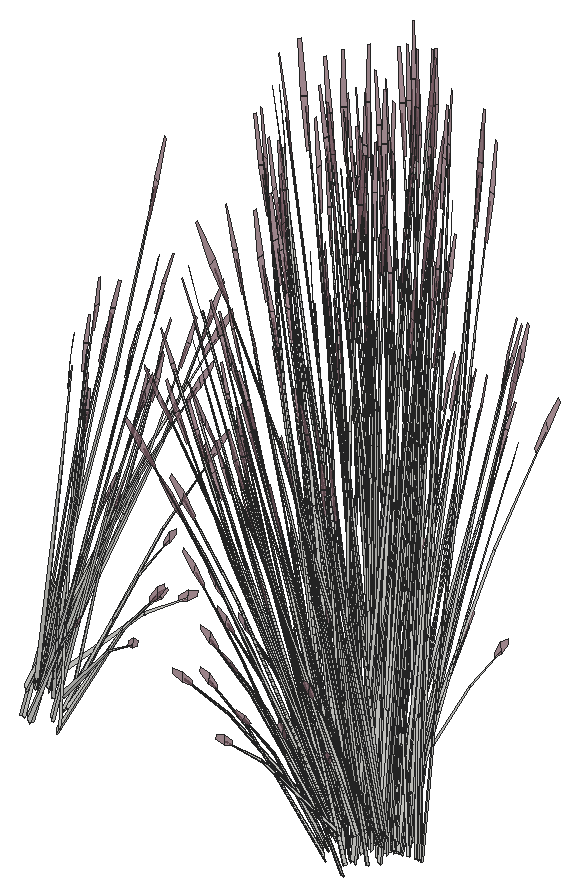
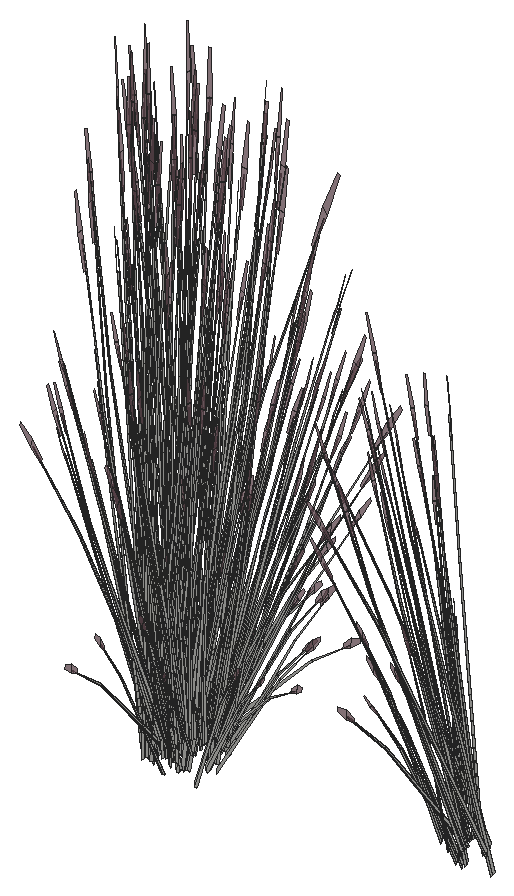
# SketchUp Ruby script. Lengths in inches.
U = 1.inch
M = Sketchup.active_model
def pt(a) = Geom::Point3d.new(a.map { |v| v * U })
def face(e, loops, mat)
  f = e.add_face(loops[0].map { |a| pt(a) })
  loops[1..].each { |l| e.add_face(l.map { |a| pt(a) }).erase! }
  f.material = f.back_material = mat if mat
  f
end
# faces: each face lists its corners as indices into pts; further lists are holes
def faces(e, pts, list, mat = nil) = list.each { |f| face(e, (f[0].is_a?(Array) ? f : [f]).map { |l| l.map { |i| pts[i] } }, mat) }
# xy, xz, yz: faces in a plane at the given z, y or x. An outline is a flat list of corners, or four numbers for a rectangle; further outlines are holes
def ring(l) = l.size == 4 ? [[l[0], l[1]], [l[2], l[1]], [l[2], l[3]], [l[0], l[3]]] : l.each_slice(2).to_a
def flat(e, list, mat, &to3) = list.each { |f| face(e, (f[0].is_a?(Array) ? f : [f]).map { |l| ring(l).map { |u, v| to3.(u, v) } }, mat) }
def xy(e, z, list, mat = nil) = flat(e, list, mat) { |x, y| [x, y, z] }
def xz(e, y, list, mat = nil) = flat(e, list, mat) { |x, z| [x, y, z] }
def yz(e, x, list, mat = nil) = flat(e, list, mat) { |y, z| [x, y, z] }
def lines(e, pts, list) = list.each { |a, b| e.add_line(pt(pts[a]), pt(pts[b])) }
# prism: a flat outline (further loops are holes) pulled along v
def prism(e, loops, v, mat = nil)
  f = face(e, loops, mat); d = Geom::Vector3d.new(v.map { |x| x * U })
  f.pushpull(f.normal.samedirection?(d) ? d.length : -d.length)
end
def box(e, o, s, mat = nil) = prism(e, [[o, [o[0] + s[0], o[1], o[2]], [o[0] + s[0], o[1] + s[1], o[2]], [o[0], o[1] + s[1], o[2]]]], [0, 0, s[2]], mat)
def at(x, y, z, deg = 0) = Geom::Transformation.translation(pt([x, y, z])) * Geom::Transformation.rotation(ORIGIN, Z_AXIS, deg.degrees)
def axes(o, x, y, z) = Geom::Transformation.new([*x, 0, *y, 0, *z, 0, *pt(o).to_a, 1])
def part(name) = M.definitions.add(name)
# library, detail: a bought-in or finely detailed component or shape, given as its bounding box
def library(name, o, s) = part(name).tap { |d| box(d.entities, o, s) }
def detail(e, o, s) = box(e.add_group.entities, o, s)
def put(e, d, t, mat = nil) = e.add_instance(d, t).tap { |i| i.material = mat if mat }
def group(e, t, mat = nil) = e.add_group.tap { |g| g.transformation = t; g.material = mat if mat }.entities
root = M.entities
M.materials.add("LightPink_Translucent").color = [144, 107, 117]
M.materials["LightPink_Translucent"].alpha = 0.75
c1 = part("blade")
p = [[2.15,0.21,22],[0,0.17,0],[0.09,0.45,0],[2.18,0.31,22],[2.29,0.31,22],[0.38,0.45,0],
  [2.48,0.24,33],[2.49,0.24,33],[2.48,0.22,33]]
faces(c1.entities,p,[[0,1,2,3],[4,5,2,3],[6,3,4,7],[8,0,3,6]])
c2 = part("seeds")
p = [[0.3,-0.1,1.38],[-0.01,-0.03,1.59],[-0.01,-0.03,0.03],[0.14,-0.07,-0.07],[0.29,-0.03,3],[0.15,0.01,3.11]]
faces(c2.entities,p,[[0,1,2,3],[1,0,4,5]],"LightPink_Translucent")
c3 = part("blade with seeds")
put(c3.entities,c1,at(0,0,0))
put(c3.entities,c2,axes([2.4,0.25,30.99],[1.5799,-0.05474,1.17369],[-0.12525,1.92788,0.29478],[-0.07173,-0.02425,1.56792]))
put(root,c3,axes([52.63,14.87,-2.07],[-0.14542,-0.51365,-0.03492],[0.68734,-0.11809,-0.15832],[0.14353,0.03256,0.52218]))
put(root,c3,axes([51.44,13.53,-0.95],[-0.63144,-0.17046,0.35414],[0.18417,-0.49731,-0.4572],[0.25423,-0.0456,0.87481]))
put(root,c3,axes([49.95,12.5,-3.94],[0.79037,0.10018,-0.62353],[-0.16679,0.61794,-0.16365],[0.23587,0.07488,1.37633]))
put(root,c3,axes([53.32,12.86,-3.74],[-0.47106,-0.39072,-0.06488],[0.51591,-0.35801,-0.29416],[0.14618,-0.02521,0.97024]))
put(root,c3,axes([52.24,10.875,-3.23],[-0.25308,0.31105,1.1486],[-0.21753,-0.4179,0.84392],[0.20902,-0.10472,0.25299]))
put(root,c3,axes([51.93,12.26,-1.27],[0.52161,0.25698,0.0643],[-0.30368,0.36595,0.50621],[0.16723,-0.11831,0.77189]))
put(root,c3,axes([51.79,12.15,-1.27],[0.18844,0.56237,0.48003],[-0.73919,0.0976,0.3958],[0.21785,-0.13226,0.9933]))
put(root,c3,axes([49.79,13.83,-2.125],[-0.28223,-0.10528,1.71376],[0.58406,-0.44165,0.13857],[0.36402,0.19924,0.73262]))
put(root,c3,axes([53.41,12.24,-1.29],[-0.09924,-0.00464,1.77383],[-0.4121,-0.49725,-0.16761],[0.1655,-0.1635,0.31391]))
put(root,c3,axes([51.875,12.04,-1.47],[0.66138,-0.08733,-0.35414],[0.17464,0.49921,0.4572],[0.18953,-0.13408,0.87481]))
put(root,c3,axes([51.35,12.21,-1.02],[0.39688,-0.48213,-0.71045],[0.69548,0.34264,0.08574],[0.23697,-0.17468,1.00501]))
put(root,c3,axes([52.01,13.6875,-1.27],[0.27906,0.41663,0.0643],[-0.50888,0.20393,0.50621],[0.22432,-0.04024,0.77189]))
put(root,c3,axes([51.34,14.81,-1.47],[0.43232,0.38257,-0.35414],[-0.49364,0.36215,0.4572],[0.25081,0.0551,0.87481]))
put(root,c3,axes([50.85,14.85,-0.97],[0.04068,-0.62141,-0.1216],[0.77029,0.01698,-0.67495],[0.29667,0.04317,1.02557]))
put(root,c3,axes([51.71,13.7,-0.97],[-0.38229,-0.5533,-0.1216],[0.6785,-0.2719,-0.67495],[0.28593,-0.073,1.02557]))
put(root,c3,axes([51.96,13.54,-1.27],[-0.21466,0.55714,0.48003],[-0.70573,-0.19051,0.3958],[0.27753,-0.03348,0.9933]))
put(root,c3,axes([51.52,14.48,-1.28],[0.16299,-0.01033,1.74944],[0.44707,-0.47471,-0.27667],[0.28992,0.06266,0.14031]))
put(root,c3,axes([51.67,13.22,-1.32],[0.20584,-0.55581,-0.51099],[0.70573,0.19051,-0.3958],[0.28414,-0.05097,0.97773]))
put(root,c3,axes([53.44,13.58,-3.23],[-0.46945,0.10088,1.1486],[0.22097,-0.4169,0.84392],[0.24904,0.02853,0.25299]))
put(root,c3,axes([51.92,11.77,-3.41],[-0.27143,-0.0181,1.43002],[-0.27808,-0.48551,-0.30754],[0.33346,-0.13735,0.61141]))
put(root,c3,axes([52.11,13.48,-1.47],[0.63144,0.17046,-0.35414],[-0.18417,0.49731,0.4572],[0.25423,-0.0456,0.87481]))
put(root,c3,axes([50.89,14.55,-1.02],[0.75952,0.01471,-0.71045],[-0.05101,0.61953,0.08574],[0.32177,0.06538,1.00501]))
put(root,c3,axes([52.43,13.38,-4.02],[-0.48937,0.07333,1.41583],[-0.07789,-0.58369,0.08104],[0.34275,-0.08835,0.80566]))
put(root,c3,axes([52.96,13,-4.51],[-0.03971,-0.09277,1.76342],[0.27541,-0.54264,-0.26939],[0.27782,-0.00781,0.30037]))
put(root,c3,axes([53.23,15.34,-1.29],[-0.0687,-0.05349,1.77383],[0.15029,-0.57341,-0.16761],[0.27062,-0.03664,0.31391]))
put(root,c3,axes([50.38,12.86,-2.125],[-0.31515,0.01384,1.71376],[0.20907,-0.5998,0.13857],[0.44912,0.0371,0.73262]))
put(root,c3,axes([51.54,13.43,-1.02],[0.66765,-0.26986,-0.71045],[0.37208,0.55551,0.08574],[0.32259,-0.0631,1.00501]))
put(root,c3,axes([53.78,12.83,-1.28],[0.10543,-0.09307,1.74944],[-0.13495,-0.57092,-0.27667],[0.26455,-0.10825,0.14031]))
put(root,c3,axes([52.56,14.25,-3.41],[-0.18299,-0.15028,1.43002],[0.23809,-0.49714,-0.30754],[0.37023,0.06735,0.61141]))
put(root,c3,axes([77.75,12.17,-2.125],[0.31515,-0.01384,1.71376],[-0.20907,0.5998,0.13857],[-0.44912,-0.0371,0.73262]))
put(root,c3,axes([77.89,13.23,-2.125],[0.26363,-0.12925,1.71376],[0.22195,0.59723,0.13857],[-0.41388,0.13498,0.73262]))
put(root,c3,axes([77.0625,14.24,-3.41],[0.26405,0.05016,1.43002],[0.17019,0.51235,-0.30754],[-0.35868,0.0959,0.61141]))
put(root,c3,axes([79.4,12.6,-2.66],[0.21597,-0.08839,1.77064],[0.07448,0.61717,0.13857],[-0.4678,0.08189,0.63284]))
put(root,c3,axes([77.08,13.02,-1.28],[-0.12407,0.07933,1.74944],[0.01055,0.57963,-0.27667],[-0.2844,0.07538,0.14031]))
put(root,c3,axes([78.7,11.61,-1.02],[-0.75952,-0.01471,-0.71045],[0.05101,-0.61953,0.08574],[-0.32177,-0.06538,1.00501]))
put(root,c3,axes([78.08,11.76,-3.41],[0.14835,0.17012,1.43002],[-0.34183,0.46242,-0.30754],[-0.351,-0.11053,0.61141]))
put(root,c3,axes([77.48,12.6875,-1.47],[-0.63144,-0.17046,-0.35414],[0.18417,-0.49731,0.4572],[-0.25423,0.0456,0.87481]))
put(root,c3,axes([78.35,11.21,-2.125],[0.28223,0.10528,1.71376],[-0.58406,0.44165,0.13857],[-0.36402,-0.19924,0.73262]))
put(root,c3,axes([75.7,13.6,-1.29],[0.09697,0.01639,1.77383],[0.29997,0.53988,-0.16761],[-0.1985,0.1417,0.31391]))
put(root,c3,axes([77.91,12.94,-1.32],[-0.20584,0.55581,-0.51099],[-0.70573,-0.19051,-0.3958],[-0.28414,0.05097,0.97773]))
put(root,c3,axes([78.44,11.74,-1.32],[-0.55171,0.40476,-0.51099],[-0.48318,-0.42758,-0.3958],[-0.28031,-0.06159,0.97773]))
put(root,c3,axes([77.56,12.91,-4.51],[0.01927,0.0963,1.76342],[-0.38846,0.5029,-0.26939],[-0.27592,-0.02535,0.30037]))
put(root,c3,axes([77.67,10.6,-1.29],[0.05633,0.06098,1.77383],[-0.27155,0.54815,-0.16761],[-0.27501,0.00397,0.31391]))
put(root,c3,axes([76.51,15.32,-3.23],[0.31665,-0.27694,1.1486],[0.12495,0.43841,0.84392],[-0.22883,0.0785,0.25299]))
put(root,c3,axes([78.29,10.24,-1.28],[-0.16348,-0.00431,1.74944],[-0.52047,0.43131,-0.27667],[-0.2777,-0.08813,0.14031]))
put(root,c3,axes([77.625,12.625,-1.27],[0.21466,-0.55714,0.48003],[0.70573,0.19051,0.3958],[-0.27753,0.03348,0.9933]))
put(root,c3,axes([77.875,12.46,-0.97],[0.38229,0.5533,-0.1216],[-0.6785,0.2719,-0.67495],[-0.28593,0.073,1.02557]))
put(root,c3,axes([78.73,11.32,-0.97],[-0.04068,0.62141,-0.1216],[-0.77029,-0.01698,-0.67495],[-0.29667,-0.04317,1.02557]))
put(root,c3,axes([78.24,11.36,-1.47],[-0.43232,-0.38257,-0.35414],[0.49364,-0.36215,0.4572],[-0.25081,-0.0551,0.87481]))
put(root,c3,axes([77.57,12.48,-1.27],[-0.27906,-0.41663,0.0643],[0.50888,-0.20393,0.50621],[-0.22432,0.04024,0.77189]))
put(root,c3,axes([78.85,13.63,-2.125],[0.18977,-0.18775,1.71376],[0.47917,0.50677,0.13857],[-0.32866,0.23079,0.73262]))
put(root,c3,axes([77.71,14.12,-1.47],[-0.66138,0.08733,-0.35414],[-0.17464,-0.49921,0.4572],[-0.18953,0.13408,0.87481]))
put(root,c3,axes([77.35,15.6,-4.51],[0.10192,0.06105,1.76342],[0.17281,0.56562,-0.26939],[-0.22588,0.12062,0.30037]))
put(root,c3,axes([77.2,12.28,-3.23],[0.48508,-0.04372,1.1486],[-0.3077,0.38525,0.84392],[-0.23971,-0.05779,0.25299]))
put(root,c3,axes([77.79,14.01,-1.27],[-0.18844,-0.56237,0.48003],[0.73919,-0.0976,0.3958],[-0.21785,0.13226,0.9933]))
put(root,c3,axes([78.17,11.21,-0.91],[0.62747,-0.45094,0.53763],[0.54116,0.47889,0.4433],[-0.29439,-0.08318,1.11249]))
put(root,c3,axes([77.65,13.9,-1.27],[-0.52161,-0.25698,0.0643],[0.30368,-0.36595,0.50621],[-0.16723,0.11831,0.77189]))
put(root,c3,axes([78.71,14.09,-2.125],[0.14147,-0.21002,1.71376],[0.59349,0.43464,0.13857],[-0.26773,0.27089,0.73262]))
put(root,c3,axes([78.14,12.63,-0.95],[0.63144,0.17046,0.35414],[-0.18417,0.49731,-0.4572],[-0.25423,0.0456,0.87481]))
put(root,c3,axes([78.25,14.18,-1.32],[0.19519,0.55794,-0.51099],[-0.73919,0.0976,-0.3958],[-0.21183,0.14986,0.97773]))
put(root,c3,axes([78.46,11.21,-1.27],[0.03826,-0.46465,0.0643],[0.57772,0.01274,0.50621],[-0.2213,-0.04862,0.77189]))
put(root,c3,axes([77.1,15.18,-1.28],[-0.01889,0.12092,1.74944],[0.53598,0.42065,-0.27667],[-0.14032,0.19892,0.14031]))
put(root,c3,axes([80.1,13.78,-3.94],[-0.79037,-0.10018,-0.62353],[0.16679,-0.61794,-0.16365],[-0.23587,-0.07488,1.37633]))
put(root,c3,axes([80.24,10.41,-0.57],[-0.50709,0.58578,-0.13619],[-0.73436,-0.33748,-0.75594],[-0.25527,-0.1655,1.14864]))
put(root,c3,axes([78.85,11.56,-0.95],[0.43232,0.38257,0.35414],[-0.49364,0.36215,-0.4572],[-0.25081,-0.0551,0.87481]))
put(root,c3,axes([80.02,10.88,-1.02],[-0.64788,-0.29534,-0.71045],[0.46044,-0.51755,0.08574],[-0.23473,-0.17635,1.00501]))
put(root,c3,axes([79.71,10.9,-1.32],[-0.74975,0.14525,-0.51099],[-0.13115,-0.55007,-0.3958],[-0.20138,-0.15763,0.97773]))
put(root,c3,axes([79.06,14.95,-3.98],[-0.7111,-0.30552,-0.49651],[0.42504,-0.54784,0],[-0.16196,-0.06958,1.57504]))
put(root,c3,axes([78.75,10.4,-4.51],[-0.0736,0.08049,1.76342],[-0.74378,0.17355,-0.26939],[-0.17968,-0.15788,0.30037]))
put(root,c3,axes([77.9,13.78,-0.97],[0.70283,0.33692,-0.1216],[-0.40491,0.48793,-0.67495],[-0.19857,0.16961,1.02557]))
put(root,c3,axes([79.49,15.32,-3.625],[-0.47504,0.61229,0],[-0.79476,-0.34146,-0.51607],[-0.18101,-0.07777,1.63711]))
put(root,c3,axes([76.75,15.24,-0.35],[0.67048,0.16311,-0.06488],[-0.20625,0.50201,-0.29416],[-0.10966,0.07622,0.97024]))
put(root,c3,axes([78.25,13.83,-0.95],[0.66138,-0.08733,0.35414],[0.17464,0.49921,-0.4572],[-0.18953,0.13408,0.87481]))
put(root,c3,axes([78.625,16.2,-3.41],[0.23977,-0.09639,1.43002],[0.59198,0.29065,-0.30754],[-0.1762,0.25149,0.61141]))
put(root,c3,axes([78.28,10.71,-3.87],[-0.21918,0.49894,-0.03893],[-0.6746,-0.15348,-0.17649],[-0.10242,-0.08161,0.58215]))
put(root,c3,axes([80.04,9.02,-1.29],[-0.01417,0.07324,1.77383],[-0.6991,0.2658,-0.16761],[-0.20573,-0.13587,0.31391]))
put(root,c3,axes([79.29,10.08,-3.41],[-0.04601,0.19989,1.43002],[-0.67263,0.16733,-0.30754],[-0.15723,-0.25836,0.61141]))
put(root,c3,axes([79.51,10.6,-2.125],[0.17368,0.19618,1.71376],[-0.80256,0.16516,0.13857],[-0.18139,-0.30799,0.73262]))
put(root,c3,axes([80.99,13.87,-3.33],[-0.76714,0.40567,-0.29095],[-0.51013,-0.57321,-0.50002],[-0.18927,-0.05821,1.59708]))
put(root,c3,axes([78.87,15.15,-1.27],[-0.54105,-0.41691,0.48003],[0.57458,-0.35956,0.3958],[-0.0998,0.1956,0.9933]))
put(root,c3,axes([79.79,10.49,-1.47],[-0.11735,-0.49217,-0.35414],[0.67083,-0.12996,0.4572],[-0.18018,-0.14104,0.87481]))
put(root,c3,axes([77.92,12.99,-3.625],[-0.95008,0,0],[0,-0.68292,-0.51607],[0,-0.15554,1.63711]))
put(root,c3,axes([79.26,14.72,-3.97],[-0.17848,-0.53243,-0.30978],[0.70886,-0.15119,0.30978],[-0.1429,-0.0614,1.38974]))
put(root,c3,axes([78.67,15.11,-1.27],[-0.62439,-0.02847,0.0643],[0.01712,-0.42991,0.50621],[-0.06534,0.16468,0.77189]))
put(root,c3,axes([78.87,15.28,-1.47],[-0.5141,0.32171,-0.35414],[-0.48666,-0.36734,0.4572],[-0.07405,0.18664,0.87481]))
put(root,c3,axes([81.5,14.3125,-3.94],[-0.51177,0.45928,-0.62353],[-0.63575,-0.41646,-0.16365],[-0.20507,0.11457,1.37633]))
put(root,c3,axes([80.19,10.89,-0.95],[0.11735,0.49217,0.35414],[-0.67083,0.12996,-0.4572],[-0.18018,-0.14104,0.87481]))
put(root,c3,axes([77.04,16.42,-1.29],[0.0862,-0.03689,1.77383],[0.71245,0.24539,-0.16761],[-0.01674,0.20431,0.31391]))
put(root,c3,axes([78.66,12.81,-3.67],[-0.70674,0.51372,0.30756],[-0.70717,-0.50832,-0.36492],[-0.02468,-0.14589,1.64885]))
put(root,c3,axes([81.57,14.22,-2.67],[0.65659,0.2464,1.51261],[-0.64324,0.53082,0.59816],[-0.28812,-0.31461,1.26806]))
put(root,c3,axes([79.0625,9.76,-3.23],[0.39634,0.21267,1.1486],[-0.57721,0.12784,0.84392],[-0.1235,-0.16344,0.25299]))
put(root,c3,axes([81.85,14.05,-3.54],[-0.74193,-0.49181,-0.25192],[0.6243,-0.55226,0.5513],[-0.19979,0.05753,1.68216]))
put(root,c3,axes([80.51,13.58,-3.79],[-0.45644,-0.51287,-0.44739],[0.69137,-0.36116,0.21531],[-0.14771,-0.06346,1.43643]))
put(root,c3,axes([79.21,14.9375,-0.66],[-0.01977,0.56521,-0.7886],[-0.83252,-0.03796,0.09517],[-0.08786,0.23945,1.11556]))
put(root,c3,axes([79.2,16.53,-3.23],[-0.01966,-0.36332,1.1486],[0.49135,0.25914,0.84392],[-0.09663,0.17317,0.25299]))
put(root,c3,axes([79.89,10.31,-0.91],[0.84639,-0.15705,0.53763],[0.14689,0.61608,0.4433],[-0.19906,-0.18157,1.11249]))
put(root,c3,axes([81.48,13.95,-3.79],[-0.82508,0.03772,-0.44739],[-0.07462,-0.62614,0.21531],[-0.14771,0.06346,1.43643]))
put(root,c3,axes([80.08,10.45,-1.27],[0.34533,-0.38816,0.0643],[0.49176,0.22599,0.50621],[-0.15898,-0.12445,0.77189]))
put(root,c3,axes([79.9,15,-3.52],[0.7111,0.30552,0.49651],[-0.42504,0.54784,0],[-0.16196,-0.06958,1.57504]))
put(root,c3,axes([78.94,15.73,-2.64],[0.01669,-0.31544,1.54345],[0.75083,0.16661,0.21329],[-0.06506,0.33618,0.72882]))
put(root,c3,axes([80.57,13.875,-3.5625],[0.20138,-0.72405,-0.23429],[0.95485,0.12621,0.51271],[-0.16685,-0.09999,1.5644]))
put(root,c3,axes([80.92,14.05,-3.38],[-0.14658,0.54532,0.1448],[-0.71613,-0.09466,-0.41347],[-0.13033,-0.05599,1.26744]))
put(root,c3,axes([80.84,9.3,-1.28],[-0.11621,-0.08567,1.74944],[-0.77555,0.05431,-0.27667],[-0.12378,-0.20491,0.14031]))
put(root,c3,axes([82.35,15.57,-3.98],[-0.7111,0.30552,-0.49651],[-0.42504,-0.54784,0],[-0.16196,0.06958,1.57504]))
put(root,c3,axes([78.14,12.52,-3.98],[0,-0.61104,-0.49651],[0.85008,0,0],[0,-0.13917,1.57504]))
put(root,c3,axes([78.5,13.09,-3.52],[0,0.61104,0.49651],[-0.85008,0,0],[0,-0.13917,1.57504]))
put(root,c3,axes([82.39,15.4,-3.81],[-0.46912,-0.61443,-0.05142],[0.79476,-0.34146,0.51607],[-0.19584,0.0585,1.6363]))
put(root,c3,axes([79.38,15.125,-1],[0.54391,0.41056,-0.5672],[-0.57458,0.35956,-0.43934],[-0.08276,0.2086,1.08528]))
put(root,c3,axes([82.18,15.32,-3.97],[-0.70886,-0.15119,-0.30978],[0.17848,-0.53243,0.30978],[-0.1429,0.0614,1.38974]))
put(root,c3,axes([79.14,14.82,-0.95],[0.5141,-0.32171,0.35414],[0.48666,0.36734,-0.4572],[-0.07405,0.18664,0.87481]))
put(root,c3,axes([80.36,13.23,-3.33],[-0.85568,-0.29155,-0.29095],[0.41201,-0.61537,-0.50002],[-0.02689,-0.15109,1.59708]))
put(root,c3,axes([82.59,13.05,-3.16],[-0.02076,-0.57531,1.41272],[0.93937,0.14913,0.59816],[-0.22217,0.31481,1.3335]))
put(root,c3,axes([78.8125,14.91,-0.6],[0.83505,0.03027,-0.13498],[-0.02282,0.57322,-0.74919],[-0.05801,0.22077,1.13838]))
put(root,c3,axes([78.79,15.74,-3.18],[0.69024,-0.1082,0.06507],[0.15868,0.43593,-0.86304],[-0.04376,0.22067,0.7736]))
put(root,c3,axes([82.06,13.78,-3.33],[0.08854,0.69723,-0.29095],[-0.92215,0.04216,-0.50002],[-0.16238,0.09287,1.59708]))
put(root,c3,axes([79.97,12.61,-3.9],[-0.31203,-0.62659,-0.69835],[0.89884,-0.22566,-0.18329],[-0.03449,-0.21218,1.54149]))
put(root,c3,axes([82.02,10.62,-0.97],[-0.74352,0.28449,-0.1216],[-0.36538,-0.50492,-0.67495],[-0.0981,-0.21277,1.02557]))
put(root,c3,axes([81.38,10.64,-1.32],[-0.7469,-0.15318,-0.51099],[0.25601,-0.52518,-0.3958],[-0.06849,-0.21144,0.97773]))
put(root,c3,axes([80,14.54,-2.125],[-0.0186,-0.23452,1.71376],[0.80601,0.15558,0.13857],[-0.04985,0.33422,0.73262]))
put(root,c3,axes([78.5,12.54,-3.97],[0.53038,-0.38124,-0.30978],[0.53038,0.38124,0.30978],[0,-0.1228,1.38974]))
put(root,c3,axes([80.89,10.07,-3.87],[-0.52505,0.35054,-0.03893],[-0.48109,-0.38392,-0.17649],[-0.03387,-0.10878,0.58215]))
put(root,c3,axes([80.68,13.53,-3.64],[0.96033,0.12874,0.45755],[-0.19544,0.7271,0.17955],[-0.14034,-0.07021,1.58856]))
put(root,c3,axes([80.43,13.4,-3.28],[-0.36864,0.55059,0.44739],[-0.76598,-0.26498,-0.21531],[0,-0.12692,1.43643]))
put(root,c3,axes([81.65,10.74,-1.02],[-0.36264,-0.49684,-0.71045],[0.74649,-0.27689,0.08574],[-0.0848,-0.24006,1.00501]))
put(root,c3,axes([80.17,14.6875,-3.53],[0.81646,-0.16218,0.17642],[0.20161,0.60355,0.35086],[-0.07282,-0.08794,1.60407]))
put(root,c3,axes([81.22,14.78,-3.8],[-0.76598,-0.27433,0],[0.36864,-0.57001,0],[0,0,1.62707]))
put(root,c3,axes([81.79,10.82,-0.95],[-0.22906,0.4699,0.35414],[-0.66828,-0.13705,-0.4572],[-0.06128,-0.18919,0.87481]))
put(root,c3,axes([82.99,15.47,-3.625],[0.47504,0.61229,0],[-0.79476,0.34146,-0.51607],[-0.18101,0.07777,1.63711]))
put(root,c3,axes([80.57,15.73,-0.9375],[-0.74868,-0.15974,0.53283],[0.25601,-0.52518,0.43934],[0.04499,0.20653,1.10256]))
put(root,c3,axes([80.375,15.77,-1.27],[-0.55987,0.20767,0.0643],[-0.27403,-0.37869,0.50621],[0.05407,0.16693,0.77189]))
put(root,c3,axes([82.6,14.72,-3.53],[0.21949,-0.60727,0.17642],[0.8032,0.17185,0.35086],[-0.13875,0.00296,1.60407]))
put(root,c3,axes([82.23,13.92,-3.38],[0.56134,0.36712,0.1448],[-0.46823,0.41419,-0.41347],[-0.13033,0.05599,1.26744]))
put(root,c3,axes([82.03,13.46,-3.7],[-0.70674,-0.52593,-0.06131],[0.70717,-0.52625,0],[-0.02468,-0.01837,1.75571]))
put(root,c3,axes([82.21,13.65,-3.28],[0.82508,-0.03772,0.44739],[0.07462,0.62614,-0.21531],[-0.14771,0.06346,1.43643]))
put(root,c3,axes([82.41,15.09,-3.67],[0.95122,0.19861,0.30756],[-0.23797,0.7099,-0.36492],[-0.15744,0.08885,1.64885]))
put(root,c3,axes([81.03,9.64,-4.51],[-0.12744,0.02202,1.76342],[-0.70477,-0.24781,-0.26939],[0.01183,-0.2067,0.30037]))
put(root,c3,axes([82.82,15.05,-3.52],[0.7111,-0.30552,0.49651],[0.42504,0.54784,0],[-0.16196,0.06958,1.57504]))
put(root,c3,axes([81.72,10.32,-1.47],[0.22906,-0.4699,-0.35414],[0.66828,0.13705,0.4572],[-0.06128,-0.18919,0.87481]))
put(root,c3,axes([80.6,12.86,-3.64],[0.33034,0.68327,0.45755],[-0.94388,0.2376,0.17955],[0.01154,-0.12555,1.58856]))
put(root,c3,axes([80.45,12.77,-3.79],[0.36864,-0.55059,-0.44739],[0.76598,0.26498,0.21531],[0,-0.12692,1.43643]))
put(root,c3,axes([81.39,14.55,-3.8],[-0.24791,-0.5268,0],[0.70791,-0.18448,0],[0,0,1.54371]))
put(root,c3,axes([80.49,15.66,-4.51],[0.12297,-0.03325,1.76342],[0.73967,0.18301,-0.26939],[0.02163,0.20626,0.30037]))
put(root,c3,axes([80.66,15.84,-1.47],[-0.22906,0.4699,-0.35414],[-0.66828,-0.13705,0.4572],[0.06128,0.18919,0.87481]))
put(root,c3,axes([82.39,13.51,-3.79],[-0.36864,0.55059,-0.44739],[-0.76598,-0.26498,0.21531],[0,0.12692,1.43643]))
put(root,c3,axes([82,10.39,-1.27],[0.55987,-0.20767,0.0643],[0.27403,0.37869,0.50621],[-0.05407,-0.16693,0.77189]))
put(root,c3,axes([80.18,16.68,-1.28],[0.09631,0.0984,1.74944],[0.77725,0.03866,-0.27667],[0.07816,0.217,0.14031]))
put(root,c3,axes([83.85,13.17,-3.53],[-0.59697,-0.44509,0.17642],[0.60159,-0.4317,0.35086],[-0.06593,0.0909,1.60407]))
put(root,c3,axes([81.79,12.92,-3.79],[0,-0.70701,0],[0.95008,0,0],[0,0,1.79456]))
put(root,c3,axes([81.8,10.43,-1.27],[0.74868,0.15974,0.48003],[-0.25601,0.52518,0.3958],[-0.04499,-0.20653,0.9933]))
put(root,c3,axes([80.91,13.04,-3.57],[0.8561,0.29616,0.24065],[-0.41201,0.61537,0.50002],[0,-0.14185,1.60543]))
put(root,c3,axes([82.27,13.2,-3.71],[0,0.70667,-0.05637],[-0.95008,0,0],[0,0.02221,1.79368]))
put(root,c3,axes([80.63,12.63,-3.28],[-0.82508,0.03772,0.44739],[-0.07462,-0.62614,-0.21531],[0.14771,-0.06346,1.43643]))
put(root,c3,axes([80.58,15.35,-0.95],[0.22906,-0.4699,0.35414],[0.66828,0.13705,-0.4572],[0.06128,0.18919,0.87481]))
put(root,c3,axes([80.24,11.56,-3.53],[-0.21949,0.60727,0.17642],[-0.8032,-0.17185,0.35086],[0.13875,-0.00296,1.60407]))
put(root,c3,axes([81.8125,14.57,-3.71],[0.33034,0.70197,-0.06012],[-0.94388,0.24598,0],[0.01154,0.02451,1.72173]))
put(root,c3,axes([79.85,10.81,-3.625],[-0.47504,-0.61229,0],[0.79476,-0.34146,-0.51607],[0.18101,-0.07777,1.63711]))
put(root,c3,axes([80.72,15.42,-1.02],[0.36264,0.49684,-0.71045],[-0.74649,0.27689,0.08574],[0.0848,0.24006,1.00501]))
put(root,c3,axes([84.54,13.64,-3.8],[-0.94962,-0.00489,-0.04976],[0,-0.68292,0.49943],[-0.02984,0.15546,1.58352]))
put(root,c3,axes([82.67,11.59,-3.53],[-0.81646,0.16218,0.17642],[-0.20161,-0.60355,0.35086],[0.07282,0.08794,1.60407]))
put(root,c3,axes([81.84,9.33,-3.23],[0.09747,0.35631,1.1486],[-0.54071,-0.19735,0.84392],[0.05818,-0.18244,0.25299]))
put(root,c3,axes([81.48,17.03,-0.35],[0.52505,-0.35054,-0.06488],[0.48109,0.38392,-0.29416],[0.03387,0.10878,0.97024]))
put(root,c3,axes([81.34,12.47,-3.64],[-0.62999,0.55453,0.45755],[-0.74845,-0.4895,0.17955],[0.15188,-0.05534,1.58856]))
put(root,c3,axes([82.41,13.34,-3.79],[0.53038,0.39469,0],[-0.53038,0.39469,0],[0,0,1.69266]))
put(root,c3,axes([82.41,12.88,-3.28],[0.36864,-0.55059,0.44739],[0.76598,0.26498,-0.21531],[0,0.12692,1.43643]))
put(root,c3,axes([82.09,14.8,-3.8],[0.76598,0.27433,0],[-0.36864,0.57001,0],[0,0,1.74954]))
put(root,c3,axes([81,15.52,-1.32],[0.7469,0.15318,-0.51099],[-0.25601,0.52518,-0.3958],[0.06849,0.21144,0.97773]))
put(root,c3,axes([80.36,15.55,-0.97],[0.74352,-0.28449,-0.1216],[0.36538,0.50492,-0.67495],[0.0981,0.21277,1.02557]))
put(root,c3,axes([82.16,12.75,-3.62],[-0.96033,-0.12874,0.49198],[0.19544,-0.7271,0.19306],[0.14034,0.07021,1.70813]))
put(root,c3,axes([84.16,9.91,-1.29],[-0.07716,0.04667,1.77383],[-0.75601,-0.15746,-0.16761],[-0.02737,-0.20368,0.31391]))
put(root,c3,axes([83.5625,11.26,-0.97],[-0.83505,-0.03027,-0.1216],[0.02282,-0.57322,-0.67495],[0.05801,-0.22077,1.02557]))
put(root,c3,axes([84.34,13.74,-3.97],[-0.53038,0.38124,-0.30978],[-0.53038,-0.38124,0.30978],[0,0.1228,1.38974]))
put(root,c3,axes([82.83,13.67,-3.91],[0.2786,0.55945,-0.69212],[-0.80253,0.20149,-0.18165],[0.03079,0.18945,1.52773]))
put(root,c3,axes([82.43,13.07,-3.79],[0.85008,0,0],[0,0.63259,0],[0,0,1.78407]))
put(root,c3,axes([83.24,11.35,-0.95],[-0.5141,0.32171,0.35414],[-0.48666,-0.36734,-0.4572],[0.07405,-0.18664,0.87481]))
put(root,c3,axes([81.62,12.375,-3.28],[-0.45644,-0.51287,0.44739],[0.69137,-0.36116,-0.21531],[0.14771,0.06346,1.43643]))
put(root,c3,axes([80.79,12.5,-3.33],[-0.08854,-0.69723,-0.29095],[0.92215,-0.04216,-0.50002],[0.16238,-0.09287,1.59708]))
put(root,c3,axes([82.73,13.01,-3.38],[0.70791,-0.1782,0.1448],[0.24791,0.50885,-0.41347],[0,0.11199,1.26744]))
put(root,c3,axes([82.99,11.04,-1.32],[-0.54391,-0.41056,-0.51099],[0.57458,-0.35956,-0.3958],[0.08276,-0.2086,0.97773]))
put(root,c3,axes([82.49,13.05,-3.33],[0.85568,0.29155,-0.29095],[-0.41201,0.61537,-0.50002],[0.02689,0.15109,1.59708]))
put(root,c3,axes([80.66,10.95,-3.97],[0.70886,0.15119,-0.30978],[-0.17848,0.53243,0.30978],[0.1429,-0.0614,1.38974]))
put(root,c3,axes([82.64,10.3125,-3.41],[-0.21597,0.12368,1.43002],[-0.64681,-0.21647,-0.30754],[0.1199,-0.26922,0.61141]))
put(root,c3,axes([84.34,13.19,-3.52],[0,-0.61104,0.49651],[0.85008,0,0],[0,0.13917,1.57504]))
put(root,c3,axes([84.71,13.76,-3.98],[0,0.61104,-0.49651],[-0.85008,0,0],[0,0.13917,1.57504]))
put(root,c3,axes([82.4375,15.61,-1.27],[-0.75571,0.14023,0.48003],[-0.13115,-0.55007,0.3958],[0.17773,0.16212,0.9933]))
put(root,c3,axes([80.5,10.71,-3.98],[0.7111,-0.30552,-0.49651],[0.42504,0.54784,0],[0.16196,-0.06958,1.57504]))
put(root,c3,axes([82.29,15.72,-1.27],[-0.34533,0.38816,0.0643],[-0.49176,-0.22599,0.50621],[0.15898,0.12445,0.77189]))
put(root,c3,axes([81.42,14.4375,-2.125],[-0.17368,-0.19618,1.71376],[0.80256,-0.16516,0.13857],[0.18139,0.30799,0.73262]))
put(root,c3,axes([81.92,12.23,-3.38],[0.14658,-0.54532,0.1448],[0.71613,0.09466,-0.41347],[0.13033,0.05599,1.26744]))
put(root,c3,axes([82.94,11.28,-3.52],[-0.7111,-0.30552,0.49651],[0.42504,-0.54784,0],[0.16196,0.06958,1.57504]))
put(root,c3,axes([83.16,11.23,-1.02],[0.01977,-0.56521,-0.71045],[0.83252,0.03796,0.08574],[0.08786,-0.23945,1.00501]))
put(root,c3,axes([82.32,14.47,-3.82],[0.79769,-0.20732,-0.19198],[0.2803,0.59721,0.00008],[0.08805,-0.02292,1.73897]))
put(root,c3,axes([82.1875,15.27,-0.95],[-0.11735,-0.49217,0.35414],[0.67083,-0.12996,-0.4572],[0.18018,0.14104,0.87481]))
